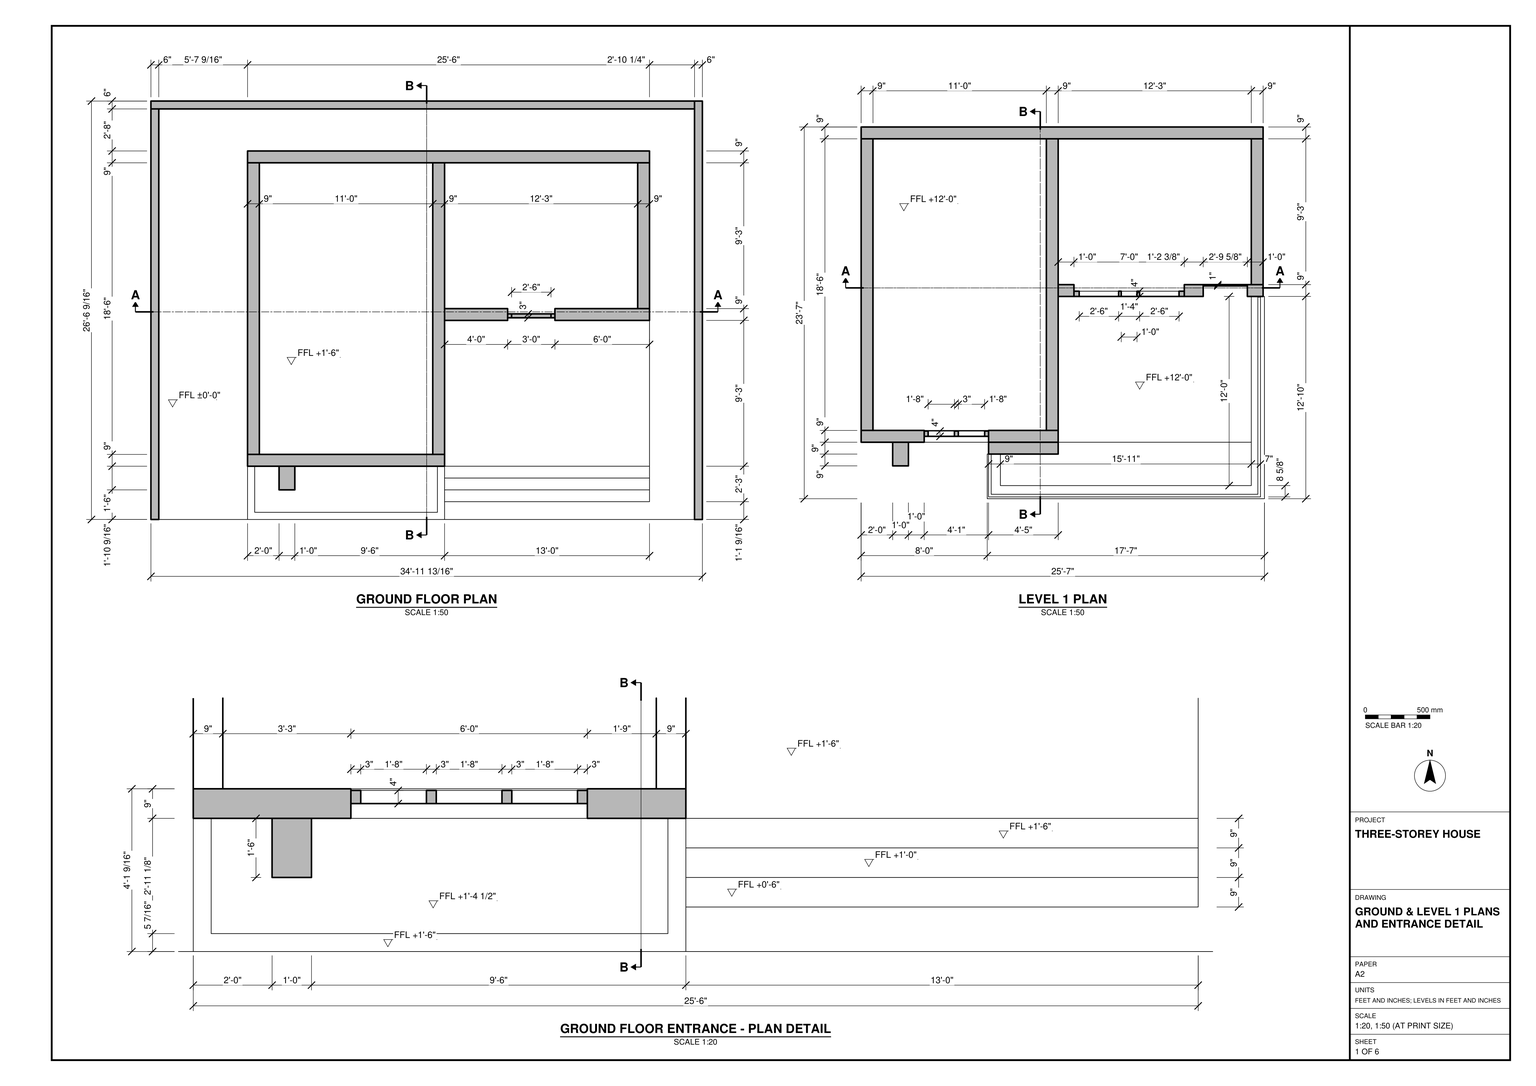
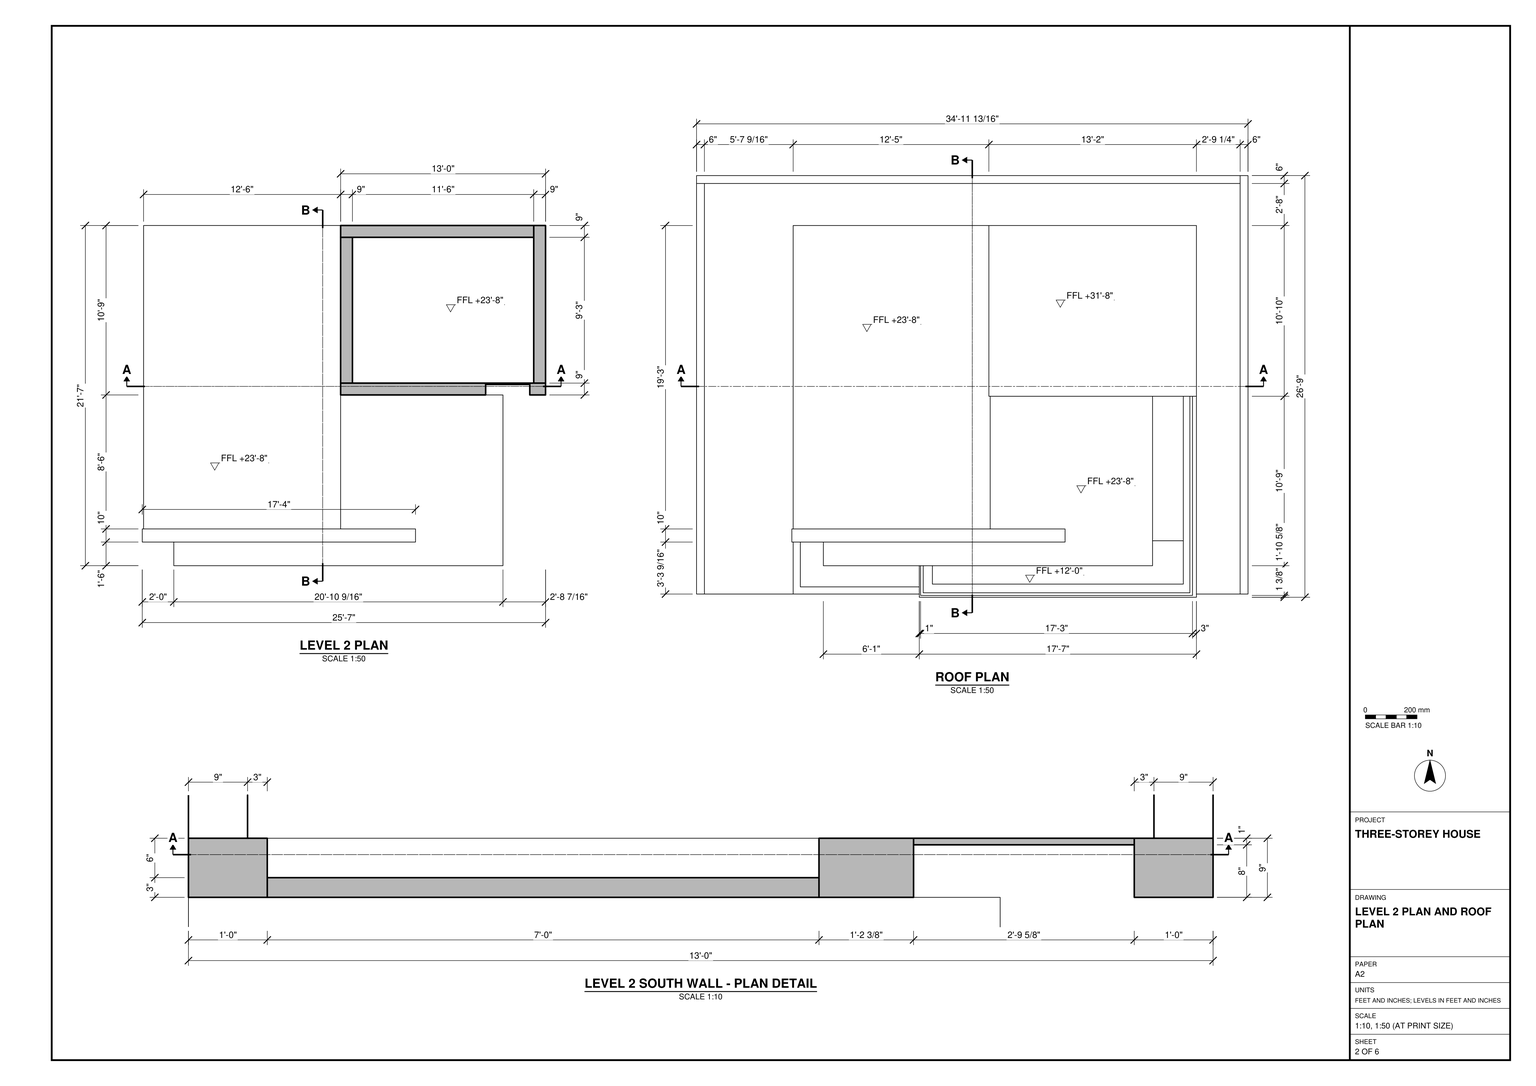
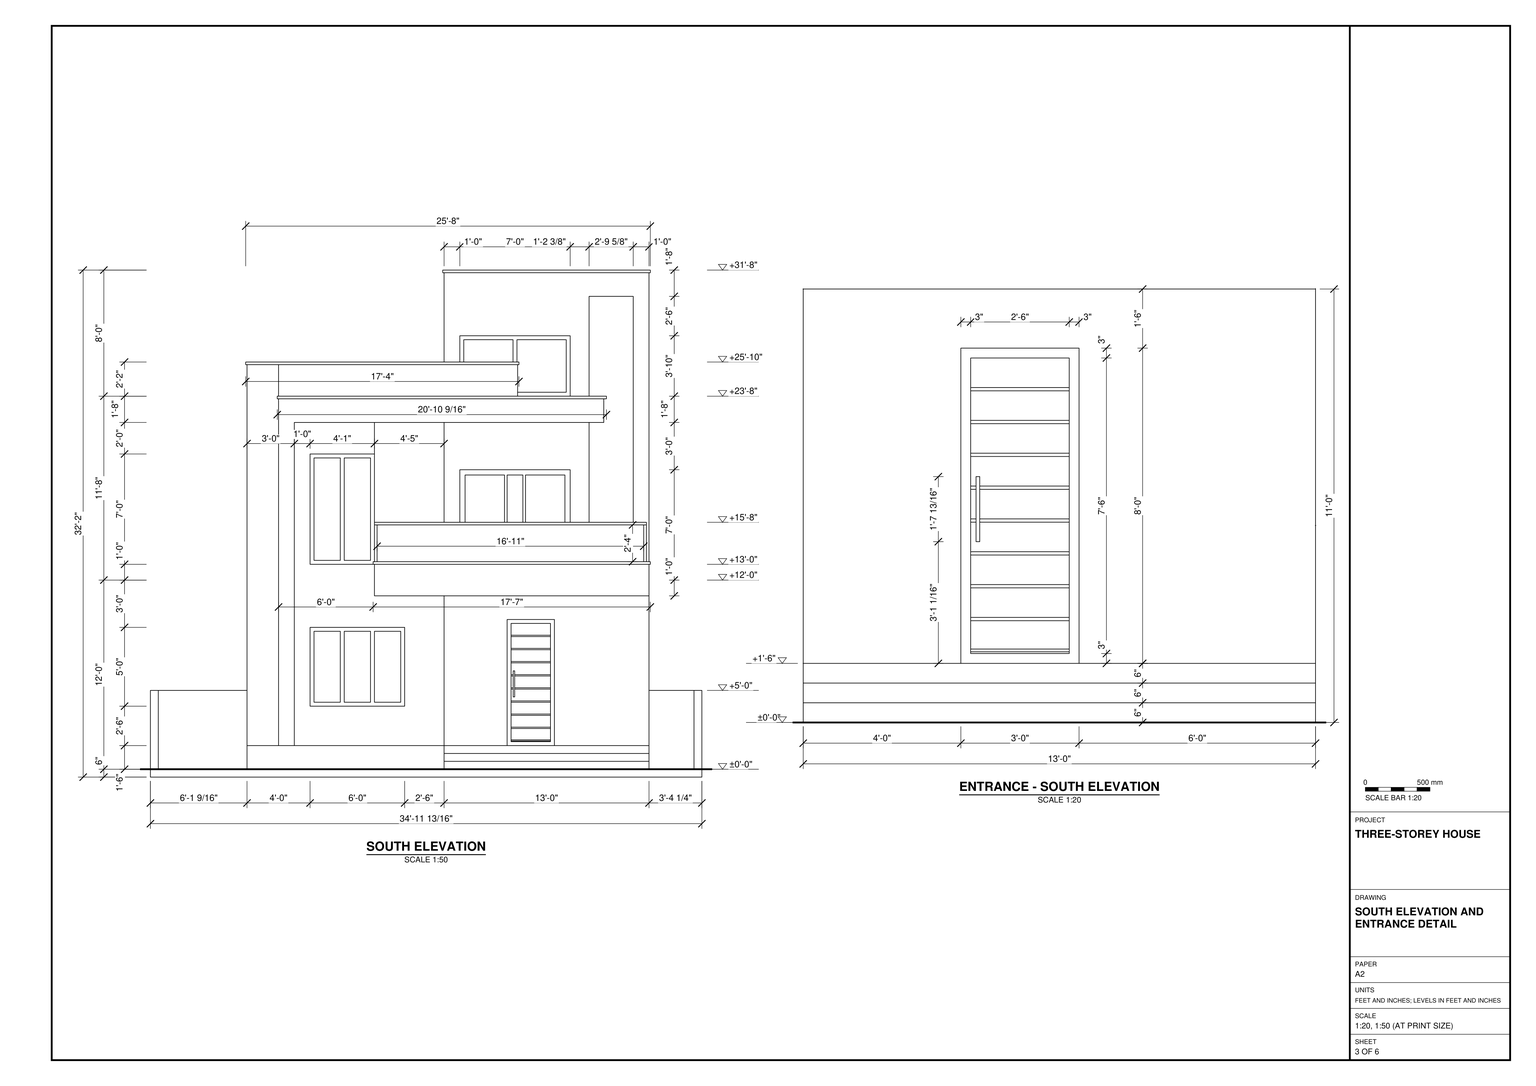
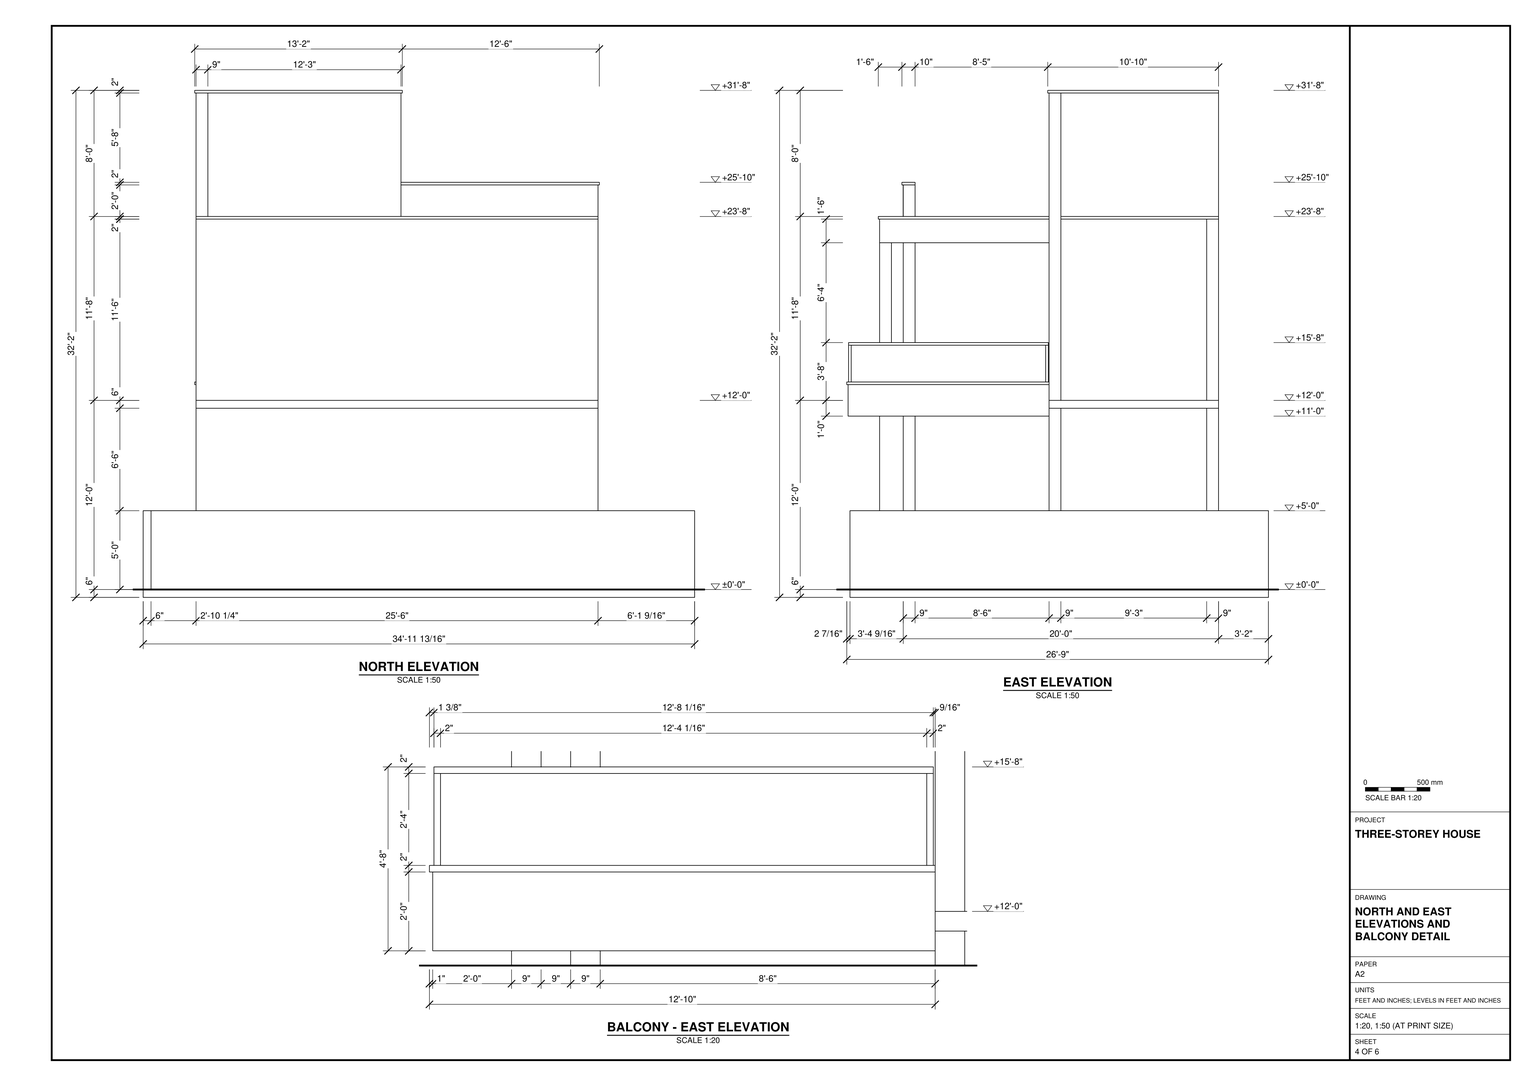
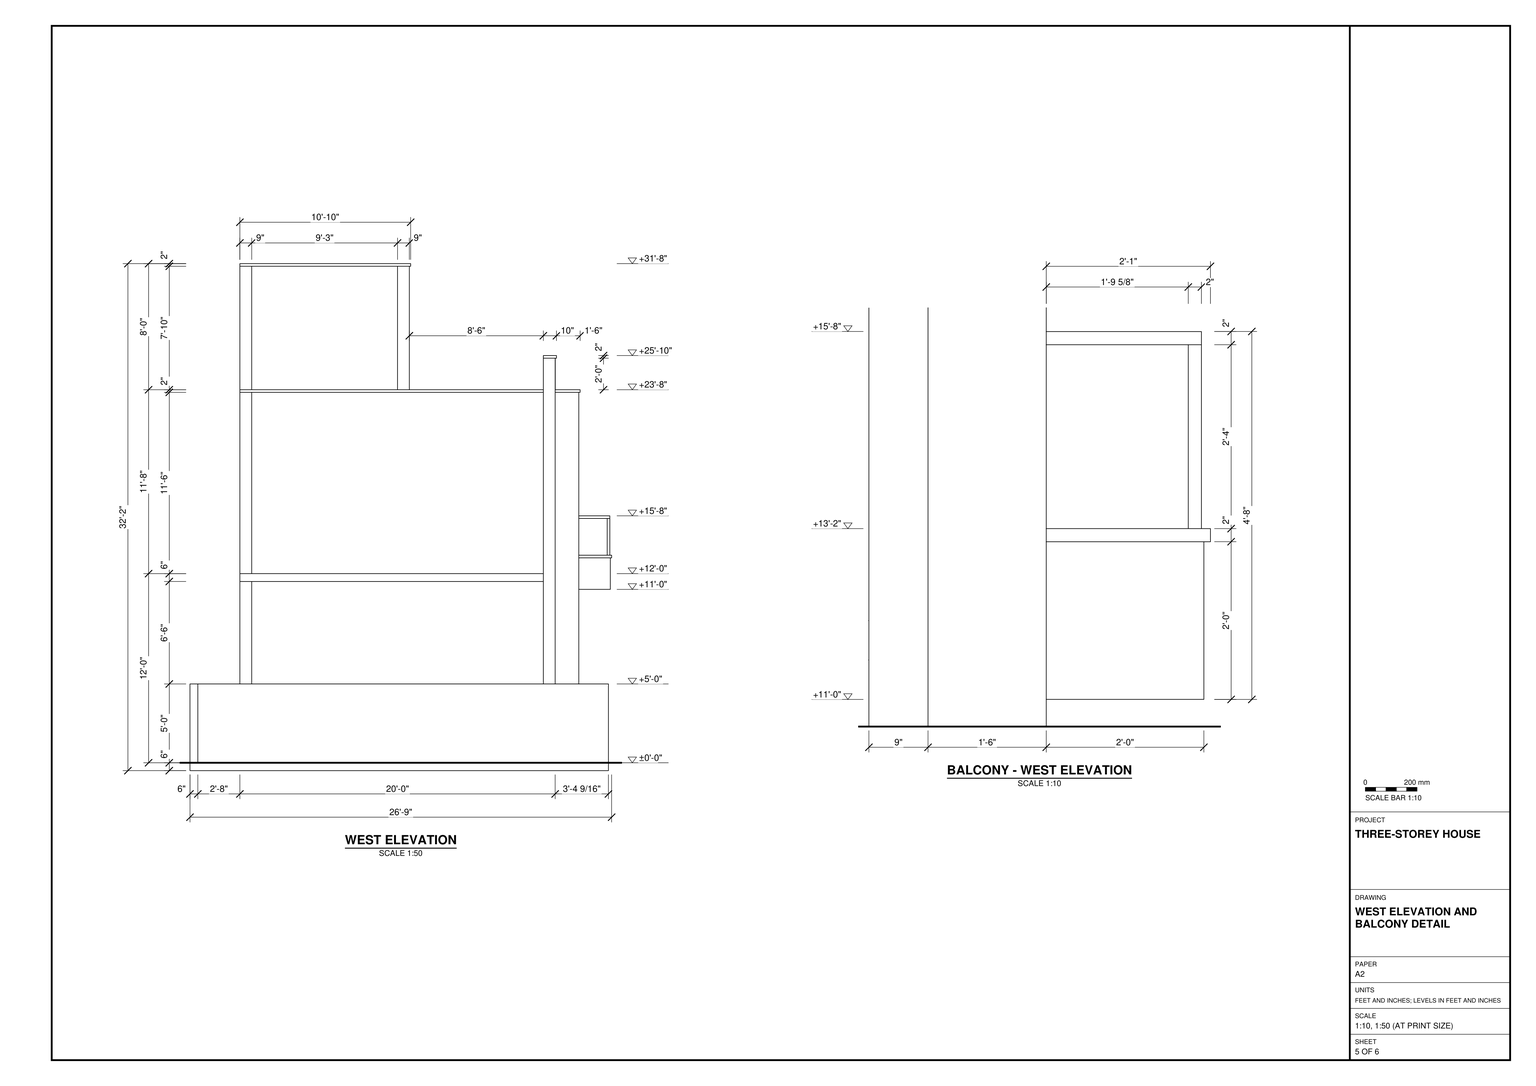
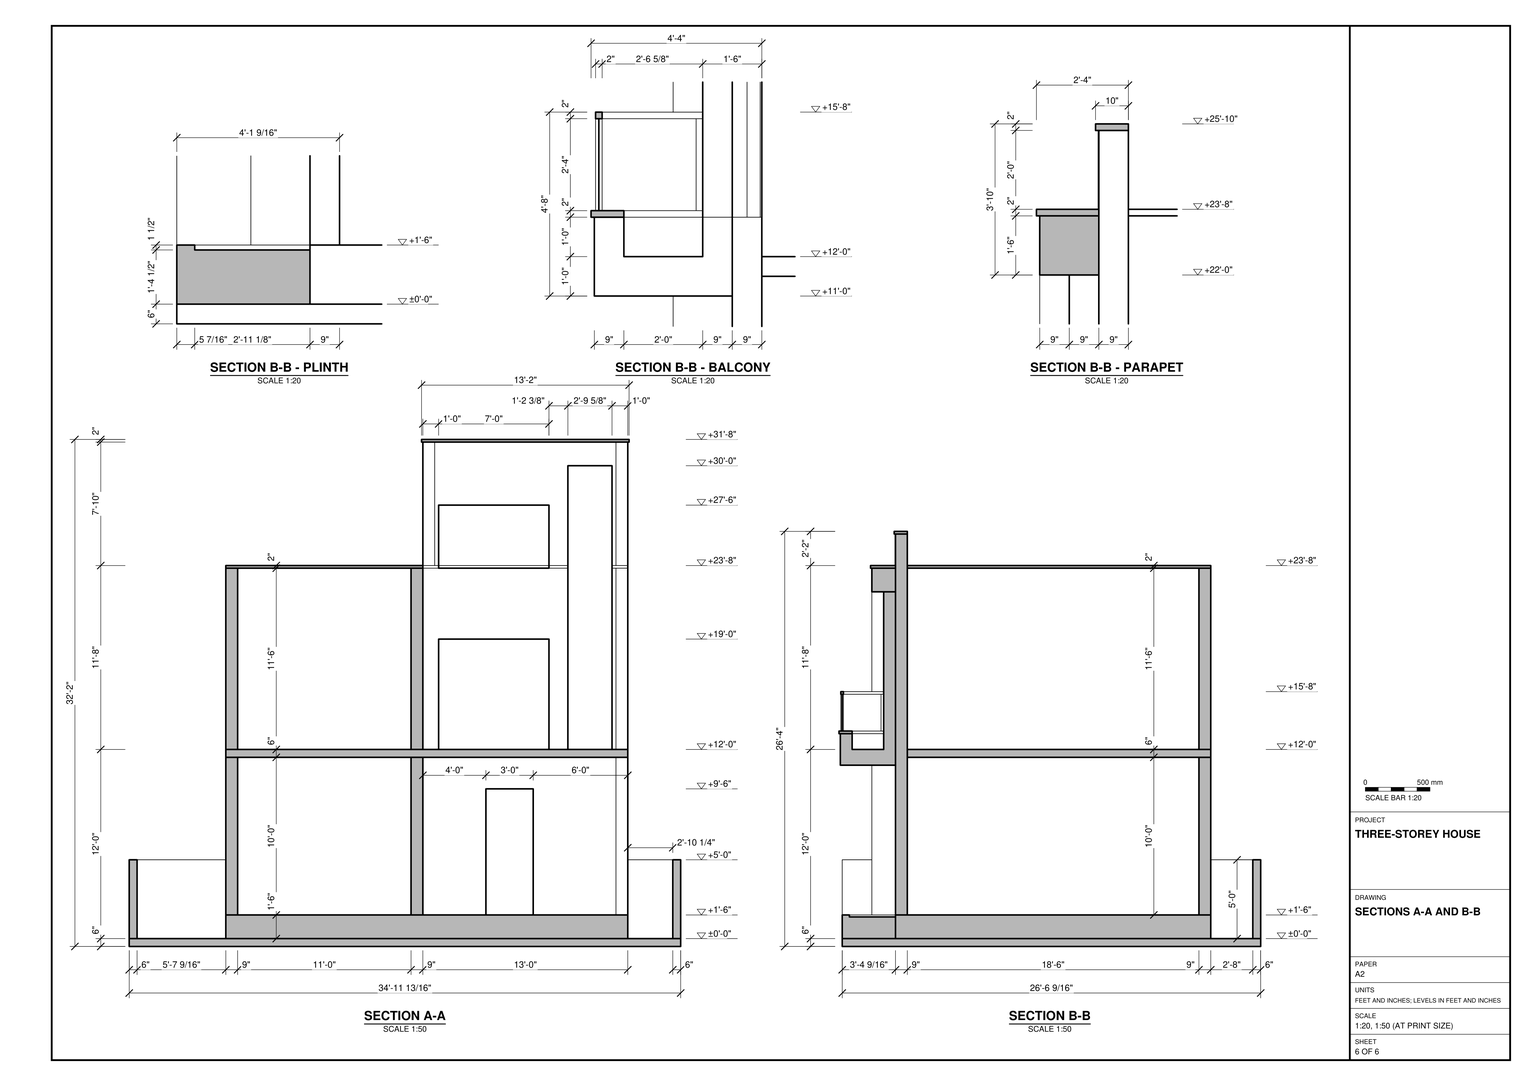
Build the three-storey house and its walled site in SketchUp using task_files/diagram_01.pdf. Work in feet and inches. Set out the complete model at 34'-11 13/16" wide, 26'-9" deep and 32'-2" high. Use ±0'-0" as the ground datum, with the upper floor levels at +12'-0" and +23'-8". Distinguish the ground datum from the raised entrance floor at +1'-6".

Start with the site base and the low walls along the sides and rear, leaving the south approach open. Set out the house walls at the thicknesses shown. On the south face, bring the left bay forward and run the entrance steps across the recessed right bay. Use the entrance detail for the door, frame and landing. Match the window openings and their divisions to the elevation. Model the projecting balcony slab and guard, the tall front frame and the offset slab edges above the balcony. At the top storey, keep the enclosed room to the rear right so the lower flat roof forms a terrace to its left and front.

Keep walls, slabs and roofs in separate groups or components. Keep each furniture or joinery piece shown separate and use components for repeated parts. Decor and loose items, if shown, may be any suitable library component. Save one SketchUp model as output_files/three_storey_house_with_a_balcony_and_roof_terrace.skp.

# SketchUp Ruby script. Lengths in inches.
U = 1.inch
M = Sketchup.active_model
def pt(a) = Geom::Point3d.new(a.map { |v| v * U })
def face(e, loops, mat)
  f = e.add_face(loops[0].map { |a| pt(a) })
  loops[1..].each { |l| e.add_face(l.map { |a| pt(a) }).erase! }
  f.material = f.back_material = mat if mat
  f
end
# faces: each face lists its corners as indices into pts; further lists are holes
def faces(e, pts, list, mat = nil) = list.each { |f| face(e, (f[0].is_a?(Array) ? f : [f]).map { |l| l.map { |i| pts[i] } }, mat) }
# xy, xz, yz: faces in a plane at the given z, y or x. An outline is a flat list of corners, or four numbers for a rectangle; further outlines are holes
def ring(l) = l.size == 4 ? [[l[0], l[1]], [l[2], l[1]], [l[2], l[3]], [l[0], l[3]]] : l.each_slice(2).to_a
def flat(e, list, mat, &to3) = list.each { |f| face(e, (f[0].is_a?(Array) ? f : [f]).map { |l| ring(l).map { |u, v| to3.(u, v) } }, mat) }
def xy(e, z, list, mat = nil) = flat(e, list, mat) { |x, y| [x, y, z] }
def xz(e, y, list, mat = nil) = flat(e, list, mat) { |x, z| [x, y, z] }
def yz(e, x, list, mat = nil) = flat(e, list, mat) { |y, z| [x, y, z] }
def lines(e, pts, list) = list.each { |a, b| e.add_line(pt(pts[a]), pt(pts[b])) }
# prism: a flat outline (further loops are holes) pulled along v
def prism(e, loops, v, mat = nil)
  f = face(e, loops, mat); d = Geom::Vector3d.new(v.map { |x| x * U })
  f.pushpull(f.normal.samedirection?(d) ? d.length : -d.length)
end
def box(e, o, s, mat = nil) = prism(e, [[o, [o[0] + s[0], o[1], o[2]], [o[0] + s[0], o[1] + s[1], o[2]], [o[0], o[1] + s[1], o[2]]]], [0, 0, s[2]], mat)
def at(x, y, z, deg = 0) = Geom::Transformation.translation(pt([x, y, z])) * Geom::Transformation.rotation(ORIGIN, Z_AXIS, deg.degrees)
def axes(o, x, y, z) = Geom::Transformation.new([*x, 0, *y, 0, *z, 0, *pt(o).to_a, 1])
def part(name) = M.definitions.add(name)
# library, detail: a bought-in or finely detailed component or shape, given as its bounding box
def library(name, o, s) = part(name).tap { |d| box(d.entities, o, s) }
def detail(e, o, s) = box(e.add_group.entities, o, s)
def put(e, d, t, mat = nil) = e.add_instance(d, t).tap { |i| i.material = mat if mat }
def group(e, t, mat = nil) = e.add_group.tap { |g| g.transformation = t; g.material = mat if mat }.entities
root = M.entities
M.materials.add("[Blacktop Old 01]").color = [132, 136, 139]
M.materials.add("[Color M09]").color = [0, 0, 0]
M.materials.add("[Grass Dark Green]").color = [106, 157, 55]
M.materials.add("[Marble Carrara Floor Tile]").color = [198, 193, 204]
M.materials.add("[Metal Aluminum Anodized]").color = [202, 209, 219]
M.materials.add("[Translucent Glass Gray]").color = [39, 162, 170]
M.materials["[Translucent Glass Gray]"].alpha = 0.5
M.materials.add("[Wood Cherry Original]").color = [152, 86, 42]
c1 = part("Group\#23")
box(c1.entities,[0,0,0],[2,2,36])
g1 = group(root,at(60,2.44,0))
box(g1,[-60,0,0],[419.8125,318.5625,6])
g2 = group(root,at(103.55,43,6),"[Marble Carrara Floor Tile]")
box(g2,[-30,0,0],[306,240,18])
g3 = group(root,at(223.55,154,24))
prism(g3,[[[48,9,0],[0,9,0],[0,9,120],[156,9,120],[156,9,0],[84,9,0],[84,9,96],[48,9,96]]],[0,-9,0])
g4 = group(root,at(103.55,43,24))
xy(g4,0,[[-30,0,120,9]])
xy(g4,30,[[18,0,90,9]])
xy(g4,90,[[18,0,90,9]])
xy(g4,138,[[18,0,67,9]])
xy(g4,222,[[18,0,67,9]])
xy(g4,266,[[120,0,176,9]])
xy(g4,290,[[-31,-1,177,0],[-31,0,-30,9],[-30,0,176,9],[176,0,177,9]])
xy(g4,292,[[-31,-1,177,9]],"[Color M09]")
xz(g4,-1,[[-31,290,177,292]],"[Color M09]")
xz(g4,0,[[[-30,0,120,0,120,266,176,266,176,290,-30,290],[18,30,90,90],[18,138,67,222]]])
xz(g4,9,[[[-30,0,-30,290,176,290,176,266,120,266,120,0],[18,30,90,90],[18,138,67,222]],[-31,290,177,292]])
yz(g4,-31,[[-1,290,9,292]],"[Color M09]")
yz(g4,-30,[[0,0,9,290]])
yz(g4,18,[[0,30,9,90],[0,138,9,222]])
yz(g4,67,[[0,138,9,222]])
yz(g4,90,[[0,30,9,90]])
yz(g4,120,[[0,0,9,266]])
yz(g4,176,[[0,266,9,290]])
yz(g4,177,[[-1,290,9,292]],"[Color M09]")
g5 = group(root,at(103.55,274,24))
box(g5,[-30,0,0],[306,9,120])
g6 = group(root,at(73.55,52,24))
box(g6,[0,0,0],[9,222,120])
g7 = group(root,at(103.55,52,144))
prism(g7,[[[-30,231,0],[276,231,0],[276,102,0],[267,102,0],[267,-9,0],[120,-9,0],[120,0,0],[-30,0,0]]],[0,0,6])
g8 = group(root,at(121.55,47.5,54),"[Color M09]")
prism(g8,[[[0,4,60],[72,4,60],[72,4,0],[0,4,0]],[[23,4,3],[23,4,57],[3,4,57],[3,4,3]],[[46,4,3],[46,4,57],[26,4,57],[26,4,3]],[[69,4,57],[49,4,57],[49,4,3],[69,4,3]]],[0,-4,0])
g9 = group(root,at(170.55,47.5,57),"[Translucent Glass Gray]")
xz(g9,0,[[0,0,20,54]])
g10 = group(root,at(147.55,47.5,57),"[Translucent Glass Gray]")
xz(g10,0,[[0,0,20,54]])
g11 = group(root,at(124.55,47.5,57),"[Translucent Glass Gray]")
xz(g11,0,[[0,0,20,54]])
g12 = group(root,at(121.55,47.5,162),"[Color M09]")
prism(g12,[[[0,4,0],[0,4,84],[49,4,84],[49,4,0]],[[23,4,3],[23,4,81],[3,4,81],[3,4,3]],[[46,4,81],[26,4,81],[26,4,3],[46,4,3]]],[0,-4,0])
g13 = group(root,at(147.55,47.5,165),"[Translucent Glass Gray]")
xz(g13,0,[[0,0,20,78]])
g14 = group(root,at(124.55,47.5,165),"[Translucent Glass Gray]")
xz(g14,0,[[0,0,20,78]])
g15 = group(root,at(97.55,25,24))
xy(g15,0,[[0,0,12,18]])
xy(g15,246,[[12,0,12,18,126,18,126,129,247.59,129,247.59,0]])
xy(g15,264,[[-1,-1,0,18],[0,-1,249.59,0],[0,0,247.59,0,247.59,129,126,129,126,18,0,18],[247.59,0,249.59,129]])
xy(g15,266,[[-1,-1,249.59,-1,249.59,129,126,129,126,18,-1,18]])
xz(g15,-1,[[-1,264,249.59,266]],"[Color M09]")
xz(g15,0,[[0,0,12,0,12,246,247.59,246,247.59,264,0,264]])
xz(g15,18,[[0,0,12,246],[0,246,12,264],[12,246,126,264],[-1,264,12,266],[12,264,126,266]])
xz(g15,129,[[126,246,247.59,264],[126,264,249.59,266]])
yz(g15,-1,[[-1,264,18,266]])
yz(g15,0,[[0,0,18,264]])
yz(g15,12,[[0,0,18,246]])
yz(g15,126,[[18,246,129,264],[18,264,129,266]])
yz(g15,247.59,[[0,246,129,264]])
yz(g15,249.59,[[-1,264,129,266]],"[Color M09]")
g16 = group(root,at(170.55,1,138))
xy(g16,0,[[0,0,0,42,53,42,53,153,209,153,209,0]])
xy(g16,6,[[53,42,200,153]])
xy(g16,12,[[9,9,200,9,200,42,53,42,53,33,9,33]])
xy(g16,24,[[-1,-1,210,0],[-1,0,0,33],[0,0,209,0,209,153,200,153,200,9,9,9,9,33,0,33],[209,0,210,153]])
xy(g16,26,[[-1,-1,210,-1,210,153,200,153,200,9,9,9,9,33,-1,33]],"[Color M09]")
xy(g16,132,[[0,33,53,42]])
xz(g16,-1,[[-1,24,210,26]],"[Color M09]")
xz(g16,0,[[0,0,209,24]])
xz(g16,9,[[9,12,200,24],[9,24,200,26]])
xz(g16,33,[[9,12,53,12,53,132,0,132,0,26,9,26],[-1,24,0,26],[0,24,9,26]])
xz(g16,42,[[0,0,53,24],[53,6,200,12],[0,24,53,132]])
xz(g16,153,[[53,0,209,6],[200,6,209,24],[200,24,210,26]])
yz(g16,-1,[[-1,24,33,26]],"[Color M09]")
yz(g16,0,[[0,0,42,24],[33,24,42,132]])
yz(g16,9,[[9,12,33,24],[9,24,33,26]])
yz(g16,53,[[42,0,153,6],[33,12,42,132]])
yz(g16,200,[[42,6,153,12],[9,12,153,24],[9,24,153,26]])
yz(g16,209,[[0,0,153,24]])
yz(g16,210,[[-1,24,153,26]],"[Color M09]")
g17 = group(root,at(214.55,52,24))
box(g17,[0,0,0],[9,222,120])
g18 = group(root,at(214.55,52,150))
box(g18,[0,0,0],[9,222,138])
g19 = group(root,at(223.55,154,150))
xy(g19,0,[[0,0,12,9],[96,0,110.4,9],[144,0,156,9]])
xy(g19,84,[[12,0,96,9]])
xy(g19,138,[[12,0,96,9]])
xy(g19,186,[[12,0,96,9]])
xy(g19,216,[[110.4,0,144,9]])
xy(g19,234,[[-1,-1,157,0],[-1,0,0,129],[0,0,156,9],[156,0,157,129],[0,9,156,129]])
xy(g19,236,[[-1,-1,157,129]],"[Color M09]")
xz(g19,-1,[[-1,234,157,236]],"[Color M09]")
xz(g19,0,[[[0,0,12,0,12,84,96,84,96,0,110.4,0,110.4,216,144,216,144,0,156,0,156,234,0,234],[12,138,96,186]]])
xz(g19,9,[[[0,0,0,234,156,234,156,0,144,0,144,216,110.4,216,110.4,0,96,0,96,84,12,84,12,0],[12,138,96,186]]])
xz(g19,129,[[-1,234,157,236]])
yz(g19,-1,[[-1,234,129,236]],"[Color M09]")
yz(g19,0,[[0,0,9,234]])
yz(g19,12,[[0,0,9,84],[0,138,9,186]])
yz(g19,96,[[0,0,9,84],[0,138,9,186]])
yz(g19,110.4,[[0,0,9,216]])
yz(g19,144,[[0,0,9,216]])
yz(g19,156,[[0,0,9,234]])
yz(g19,157,[[-1,234,129,236]],"[Color M09]")
g20 = group(root,at(103.55,274,150))
box(g20,[-30,0,0],[306,9,138])
g21 = group(root,at(271.55,156,24),"[Wood Cherry Original]")
prism(g21,[[[36,3,96],[36,3,0],[0,3,0],[0,3,96]],[[3,3,3],[33,3,3],[33,3,93],[3,3,93]]],[0,-3,0])
g22 = group(root,at(274.55,157,27),"[Wood Cherry Original]")
prism(g22,[[[30,2,0],[30,2,90],[30,-1,90],[30,-1,81],[30,0,81],[30,0,80],[30,-1,80],[30,-1,71],[30,0,71],[30,0,70],[30,-1,70],[30,-1,61],[30,0,61],[30,0,60],[30,-1,60],[30,-1,51],[30,0,51],[30,0,50],[30,-1,50],[30,-1,41],[30,0,41],[30,0,40],[30,-1,40],[30,-1,31],[30,0,31],[30,0,30],[30,-1,30],[30,-1,21],[30,0,21],[30,0,20],[30,-1,20],[30,-1,11],[30,0,11],[30,0,10],[30,-1,10],[30,-1,1.36],[30,0,1.36],[30,0,0.52],[30,0,0]]],[-30,0,0])
put(root,c1,axes([170.55,1.375,164],[1,0,0],[0,1,0],[0,0,0.77778]),"[Color M09]")
put(root,c1,axes([170.55,32,164],[1,0,0],[0,1,0],[0,0,0.77778]),"[Color M09]")
put(root,c1,axes([375.55,151.4375,164],[1,0,0],[0,1,0],[0,0,0.77778]),"[Color M09]")
put(root,c1,axes([375.55,1.375,164],[1,0,0],[0,1,0],[0,0,0.77778]),"[Color M09]")
g23 = group(root,at(171.55,3.375,164),"[Translucent Glass Gray]")
yz(g23,0,[[0,0,28.625,28]])
g24 = group(root,at(172.55,2.375,164),"[Translucent Glass Gray]")
xz(g24,0,[[0,0,203,28]])
g25 = group(root,at(170.55,1.375,192),"[Color M09]")
prism(g25,[[[0,0,0],[0,32.625,0],[2,32.625,0],[2,2,0],[205,2,0],[205,152.0625,0],[207,152.0625,0],[207,0,0]]],[0,0,2])
g26 = group(root,at(235.55,154,150),"[Color M09]")
prism(g26,[[[0,4,0],[0,4,84],[84,4,84],[84,4,0]],[[34,4,4],[34,4,80],[4,4,80],[4,4,4]],[[80,4,80],[50,4,80],[50,4,4],[80,4,4]],[[48,4,4],[48,4,80],[36,4,80],[36,4,4]]],[0,-4,0])
g27 = group(root,at(285.55,154,154),"[Translucent Glass Gray]")
xz(g27,0,[[0,0,30,76]])
g28 = group(root,at(271.55,154,154),"[Translucent Glass Gray]")
xz(g28,0,[[0,0,12,76]])
g29 = group(root,at(239.55,154,154),"[Translucent Glass Gray]")
xz(g29,0,[[0,0,30,76]])
g30 = group(root,at(333.95,162,150),"[Blacktop Old 01]")
box(g30,[0,0,0],[33.6,1,216])
g31 = group(root,at(376.55,3.375,164),"[Translucent Glass Gray]")
yz(g31,0,[[0,0,148.0625,28]])
g32 = group(root,at(73.55,52,150))
box(g32,[0,0,0],[9,222,138])
g33 = group(root,at(235.55,154,290),"[Color M09]")
prism(g33,[[[0,3,46],[84,3,46],[84,3,0],[0,3,0]],[[40.5,3,3],[40.5,3,43],[3,3,43],[3,3,3]],[[81,3,43],[43.5,3,43],[43.5,3,3],[81,3,3]]],[0,-3,0])
g34 = group(root,at(279.05,154,293),"[Translucent Glass Gray]")
xz(g34,0,[[0,0,37.5,40]])
g35 = group(root,at(238.55,154,293),"[Translucent Glass Gray]")
xz(g35,0,[[0,0,37.5,40]])
g36 = group(root,at(370.55,163,24))
box(g36,[0,0,0],[9,111,120])
g37 = group(root,at(370.55,163,150))
box(g37,[0,0,0],[9,111,138])
g38 = group(root,at(73.55,163,288))
prism(g38,[[[0,120,0],[306,120,0],[306,0,0],[150,0,0],[150,-111,0],[0,-111,0]]],[0,0,2])
g39 = group(root,at(370.55,163,290))
box(g39,[0,0,0],[9,120,94])
g40 = group(root,at(223.55,274,290))
box(g40,[0,0,0],[147,9,94])
g41 = group(root,at(223.55,163,290))
box(g41,[0,0,0],[9,111,94])
g42 = group(root,at(73.55,2.44,6))
xy(g42,0,[[0,0,150,40.56]])
xy(g42,16.5,[[5.46,5.46,144.54,40.56]],"[Grass Dark Green]")
xy(g42,18,[[0,0,150,0,150,40.56,144.54,40.56,144.54,5.46,5.46,5.46,5.46,40.56,0,40.56]])
xz(g42,0,[[0,0,150,18]])
xz(g42,5.46,[[5.46,16.5,144.54,18]])
xz(g42,40.56,[[0,0,0,18,5.46,18,5.46,16.5,144.54,16.5,144.54,18,150,18,150,0]])
yz(g42,0,[[0,0,40.56,18]])
yz(g42,5.46,[[5.46,16.5,40.56,18]])
yz(g42,144.54,[[5.46,16.5,40.56,18]])
yz(g42,150,[[0,0,40.56,18]])
g43 = group(root,at(413.8125,2.44,6))
box(g43,[0,0,0],[6,318.5625,60])
g44 = group(root,at(60,315.01,6))
box(g44,[-60,0,0],[413.8125,6,60])
g45 = group(root,at(0,2.44,6))
box(g45,[0,0,0],[6,312.5625,60])
g46 = group(root,at(97.55,42.9,290),"[Blacktop Old 01]")
box(g46,[0,0,0],[182,0.1,24])
g47 = group(root,at(223.55,16,6))
xy(g47,0,[[0,0,156,27]])
xy(g47,6,[[0,0,156,9]],"[Marble Carrara Floor Tile]")
xy(g47,12,[[0,9,156,18]],"[Marble Carrara Floor Tile]")
xy(g47,18,[[0,18,156,27]],"[Marble Carrara Floor Tile]")
xz(g47,0,[[0,0,156,6]],"[Marble Carrara Floor Tile]")
xz(g47,9,[[0,6,156,12]],"[Marble Carrara Floor Tile]")
xz(g47,18,[[0,12,156,18]],"[Marble Carrara Floor Tile]")
xz(g47,27,[[0,0,156,18]])
yz(g47,0,[[0,0,0,6,9,6,9,12,18,12,18,18,27,18,27,0]])
yz(g47,156,[[0,0,27,0,27,18,18,18,18,12,9,12,9,6,0,6]],"[Marble Carrara Floor Tile]")
g48 = group(root,at(276.18,155,61.07),"[Metal Aluminum Anodized]")
box(g48,[0,0,0],[1.125,1,19.8125])
